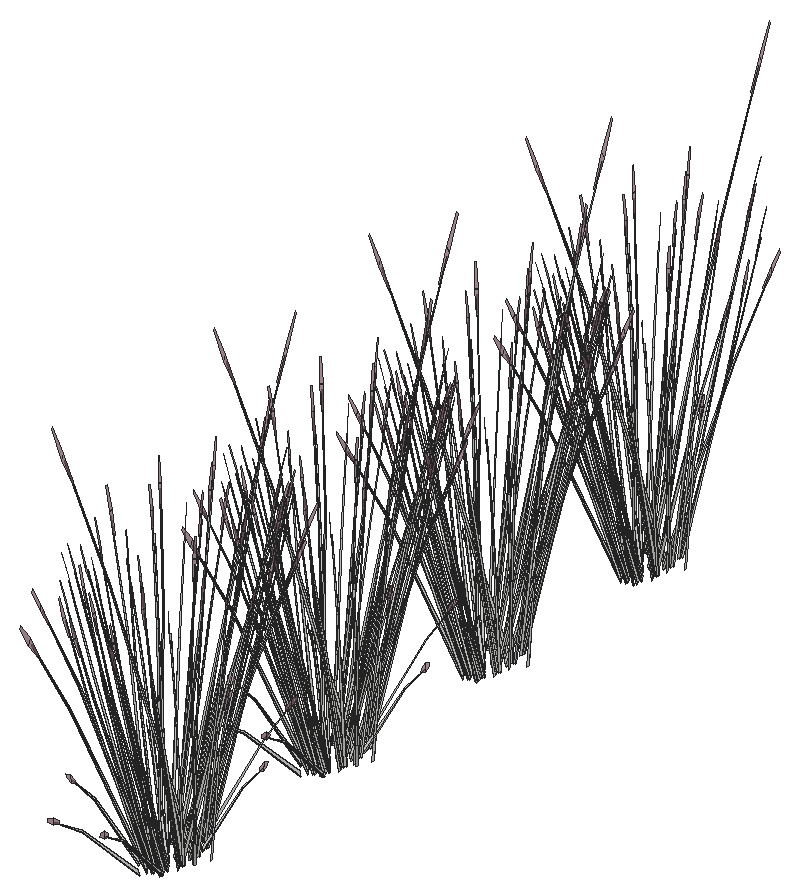
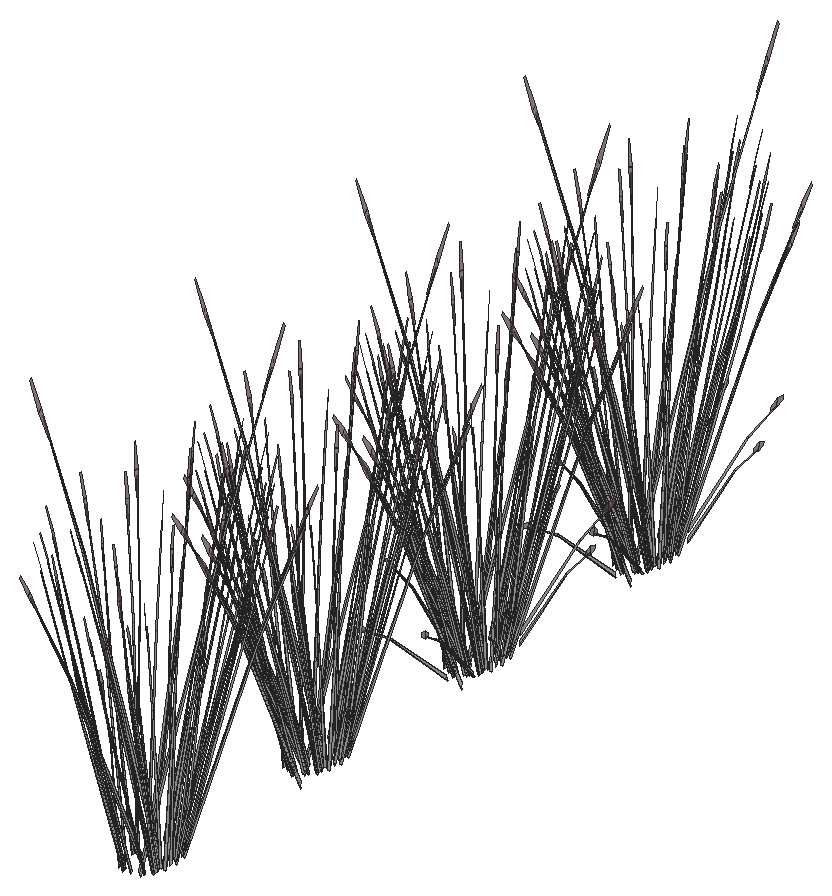
# SketchUp Ruby script. Lengths in inches.
U = 1.inch
M = Sketchup.active_model
def pt(a) = Geom::Point3d.new(a.map { |v| v * U })
def face(e, loops, mat)
  f = e.add_face(loops[0].map { |a| pt(a) })
  loops[1..].each { |l| e.add_face(l.map { |a| pt(a) }).erase! }
  f.material = f.back_material = mat if mat
  f
end
# faces: each face lists its corners as indices into pts; further lists are holes
def faces(e, pts, list, mat = nil) = list.each { |f| face(e, (f[0].is_a?(Array) ? f : [f]).map { |l| l.map { |i| pts[i] } }, mat) }
# xy, xz, yz: faces in a plane at the given z, y or x. An outline is a flat list of corners, or four numbers for a rectangle; further outlines are holes
def ring(l) = l.size == 4 ? [[l[0], l[1]], [l[2], l[1]], [l[2], l[3]], [l[0], l[3]]] : l.each_slice(2).to_a
def flat(e, list, mat, &to3) = list.each { |f| face(e, (f[0].is_a?(Array) ? f : [f]).map { |l| ring(l).map { |u, v| to3.(u, v) } }, mat) }
def xy(e, z, list, mat = nil) = flat(e, list, mat) { |x, y| [x, y, z] }
def xz(e, y, list, mat = nil) = flat(e, list, mat) { |x, z| [x, y, z] }
def yz(e, x, list, mat = nil) = flat(e, list, mat) { |y, z| [x, y, z] }
def lines(e, pts, list) = list.each { |a, b| e.add_line(pt(pts[a]), pt(pts[b])) }
# prism: a flat outline (further loops are holes) pulled along v
def prism(e, loops, v, mat = nil)
  f = face(e, loops, mat); d = Geom::Vector3d.new(v.map { |x| x * U })
  f.pushpull(f.normal.samedirection?(d) ? d.length : -d.length)
end
def box(e, o, s, mat = nil) = prism(e, [[o, [o[0] + s[0], o[1], o[2]], [o[0] + s[0], o[1] + s[1], o[2]], [o[0], o[1] + s[1], o[2]]]], [0, 0, s[2]], mat)
def at(x, y, z, deg = 0) = Geom::Transformation.translation(pt([x, y, z])) * Geom::Transformation.rotation(ORIGIN, Z_AXIS, deg.degrees)
def axes(o, x, y, z) = Geom::Transformation.new([*x, 0, *y, 0, *z, 0, *pt(o).to_a, 1])
def part(name) = M.definitions.add(name)
# library, detail: a bought-in or finely detailed component or shape, given as its bounding box
def library(name, o, s) = part(name).tap { |d| box(d.entities, o, s) }
def detail(e, o, s) = box(e.add_group.entities, o, s)
def put(e, d, t, mat = nil) = e.add_instance(d, t).tap { |i| i.material = mat if mat }
def group(e, t, mat = nil) = e.add_group.tap { |g| g.transformation = t; g.material = mat if mat }.entities
root = M.entities
M.materials.add("LightPink_Translucent").color = [144, 107, 117]
M.materials["LightPink_Translucent"].alpha = 0.75
c1 = part("blade")
p = [[2.15,0.21,22],[0,0.17,0],[0.09,0.45,0],[2.18,0.31,22],[2.29,0.31,22],[0.38,0.45,0],
  [2.48,0.24,33],[2.49,0.24,33],[2.48,0.22,33]]
faces(c1.entities,p,[[0,1,2,3],[4,5,2,3],[6,3,4,7],[8,0,3,6]])
c2 = part("seeds")
p = [[0.3,-0.1,1.38],[-0.01,-0.03,1.59],[-0.01,-0.03,0.03],[0.14,-0.07,-0.07],[0.29,-0.03,3],[0.15,0.01,3.11]]
faces(c2.entities,p,[[0,1,2,3],[1,0,4,5]],"LightPink_Translucent")
c3 = part("blade with seeds")
put(c3.entities,c1,at(0,0,0))
put(c3.entities,c2,axes([2.4,0.25,30.99],[1.5799,-0.05474,1.17369],[-0.12525,1.92788,0.29478],[-0.07173,-0.02425,1.56792]))
put(root,c3,axes([251.1,10.6,2.01],[0.05851,0.19632,1.24382],[-0.27036,0.16528,0.10057],[-0.0611,-0.3082,0.53172]))
put(root,c3,axes([251.55,9.3,2.61],[-0.03915,-0.08573,1.26972],[-0.26126,0.05435,-0.2008],[-0.0417,-0.20505,0.10183]))
put(root,c3,axes([252.72,10.35,2.61],[-0.00247,-0.12169,1.26972],[-0.20868,-0.35171,-0.2008],[0.03226,-0.2132,0.10183]))
put(root,c3,axes([251.84,10.33,2.48],[0.07716,-0.47021,-0.25703],[0.22512,0.13715,0.33183],[-0.02064,-0.18932,0.63492]))
put(root,c3,axes([252.01,10.95,2.01],[-0.04766,0.21017,1.24382],[-0.19993,-0.43493,0.10057],[0.09019,-0.27107,0.53172]))
put(root,c3,axes([251.73,10.65,2.59],[-0.25161,-0.15328,-0.37087],[0.08624,-0.52553,-0.28727],[-0.02307,-0.21159,0.70962]))
put(root,c3,axes([252.27,11.05,2.59],[-0.18323,-0.41084,-0.37087],[0.19356,-0.3598,-0.28727],[0.02788,-0.20874,0.70962]))
put(root,c3,axes([251.94,10.625,2.85],[-0.25047,0.28468,-0.08826],[-0.12309,-0.50526,-0.48986],[-0.03305,-0.21292,0.74434]))
put(root,c3,axes([252.46,11.26,2.85],[-0.2813,-0.0303,-0.08826],[0.00769,-0.57361,-0.48986],[0.01954,-0.22092,0.74434]))
put(root,c3,axes([252.44,10.9,2.48],[0.17318,-0.32193,-0.25703],[0.16394,0.36759,0.33183],[0.02494,-0.18677,0.63492]))
put(root,c3,axes([251.19,10.5,2.48],[-0.03953,-0.49251,-0.25703],[0.22598,-0.13005,0.33183],[-0.0607,-0.14114,0.63492]))
put(root,c3,axes([250.71,11.22,2.01],[0.09507,0.10535,1.24382],[-0.19675,0.44195,0.10057],[-0.12263,-0.19937,0.53172]))
put(root,c3,axes([251.17,10.91,2.59],[-0.25257,0.14535,-0.37087],[-0.04418,-0.55045,-0.28727],[-0.06784,-0.15774,0.70962]))
put(root,c3,axes([252.65,11.99,2.59],[-0.06575,-0.55831,-0.37087],[0.24901,-0.09767,-0.28727],[0.07136,-0.14996,0.70962]))
put(root,c3,axes([250.6875,10.25,2.61],[-0.05507,-0.00432,1.26972],[-0.17533,0.4316,-0.2008],[-0.09355,-0.08819,0.10183]))
put(root,c3,axes([252.77,12.39,2.85],[-0.23676,-0.33715,-0.08826],[0.1364,-0.48826,-0.48986],[0.06689,-0.16972,0.74434]))
put(root,c3,axes([251.79,14.23,1.61],[0.22119,0.24656,1.09782],[-0.21669,0.53118,0.43413],[-0.09706,-0.31482,0.92034]))
put(root,c3,axes([252.84,12.05,2.48],[0.2228,-0.08739,-0.25703],[0.05883,0.49954,0.33183],[0.06385,-0.13418,0.63492]))
put(root,c3,axes([250.67,11.37,2.48],[-0.14563,-0.38283,-0.25703],[0.16629,-0.3624,0.33183],[-0.08449,-0.05514,0.63492]))
put(root,c3,axes([253.48,12.84,2.61],[0.03552,-0.09314,1.26972],[-0.04546,-0.57131,-0.2008],[0.08912,-0.10832,0.10183]))
put(root,c3,axes([250.74,11.75,2.59],[-0.18586,0.40503,-0.37087],[-0.16277,-0.42787,-0.28727],[-0.09443,-0.06163,0.70962]))
put(root,c3,axes([250.84,11.32,2.85],[-0.0137,0.62183,-0.08826],[-0.25949,-0.017,-0.48986],[-0.09994,-0.0432,0.74434]))
put(root,c3,axes([252.78,13.71,2.85],[-0.12878,-0.55367,-0.08826],[0.22857,-0.27208,-0.48986],[0.09632,-0.07305,0.74434]))
put(root,c3,axes([252.77,13.23,2.59],[0.06934,-0.55619,-0.37087],[0.23774,0.19064,-0.28727],[0.09572,-0.051,0.70962]))
put(root,c3,axes([250.51,12.18,2.01],[0.10617,-0.01385,1.24382],[-0.07043,0.60021,0.10057],[-0.1513,-0.03712,0.53172]))
put(root,c3,axes([252.91,13.49,2.48],[0.21272,0.17057,-0.25703],[-0.06204,0.49764,0.33183],[0.08564,-0.04563,0.63492]))
put(root,c3,axes([250.41,12.7,2.48],[-0.21272,-0.17057,-0.25703],[0.06204,-0.49764,0.33183],[-0.08564,0.04563,0.63492]))
put(root,c3,axes([252.33,12.87,2.01],[-0.10617,0.01385,1.24382],[0.07043,-0.60021,0.10057],[0.1513,0.03712,0.53172]))
put(root,c3,axes([251.0625,12.61,1.62],[0.07276,-0.08845,1.2851],[0.02509,0.61759,0.10057],[-0.15759,0.08195,0.4593]))
put(root,c3,axes([250.28,13.03,2.61],[-0.0418,0.07939,1.26972],[0.00356,0.58003,-0.2008],[-0.09581,0.07543,0.10183]))
put(root,c3,axes([250.56,12.95,2.59],[-0.06934,0.55619,-0.37087],[-0.23774,-0.19064,-0.28727],[-0.09572,0.051,0.70962]))
put(root,c3,axes([250.55,12.47,2.85],[0.12878,0.55367,-0.08826],[-0.22857,0.27208,-0.48986],[-0.09632,0.07305,0.74434]))
put(root,c3,axes([253.09,14.875,2.04],[-0.04899,-0.514,-0.02534],[0.23154,-0.11817,-0.1149],[0.04835,0.03259,0.37899]))
put(root,c3,axes([252.49,14.86,2.85],[0.0137,-0.62183,-0.08826],[0.25949,0.017,-0.48986],[0.09994,0.0432,0.74434]))
put(root,c3,axes([252.72,14.49,2.61],[0.05491,-0.01034,1.26972],[0.1506,-0.47504,-0.2008],[0.09767,0.06271,0.10183]))
put(root,c3,axes([250.55,13.24,2.01],[0.08881,-0.12933,1.24382],[0.07477,0.59764,0.10057],[-0.13942,0.13507,0.53172]))
put(root,c3,axes([252.66,14.82,2.48],[0.14563,0.38283,-0.25703],[-0.16629,0.3624,0.33183],[0.08449,0.05514,0.63492]))
put(root,c3,axes([250.49,14.13,2.48],[-0.2228,0.08739,-0.25703],[-0.05883,-0.49954,0.33183],[-0.06385,0.13418,0.63492]))
put(root,c3,axes([252.13,13.84,2.01],[-0.09507,-0.10535,1.24382],[0.19675,-0.44195,0.10057],[0.12263,0.19937,0.53172]))
put(root,c3,axes([252.15,12.45,2.44],[-0.22117,-0.3177,1.00363],[0.23354,-0.49464,0.43304],[0.07136,0.29809,0.97011]))
put(root,c3,axes([250.56,13.79,2.85],[0.23676,0.33715,-0.08826],[-0.1364,0.48826,-0.48986],[-0.06689,0.16972,0.74434]))
put(root,c3,axes([251.98,15.54,2.85],[0.15252,-0.52338,-0.08826],[0.22088,0.30152,-0.48986],[0.07678,0.14787,0.74434]))
put(root,c3,axes([250.875,13.64,2.01],[0.06393,-0.18788,1.24382],[0.16142,0.50711,0.10057],[-0.11071,0.23094,0.53172]))
put(root,c3,axes([250.67,14.1875,2.59],[0.06575,0.55831,-0.37087],[-0.24901,0.09767,-0.28727],[-0.07136,0.14996,0.70962]))
put(root,c3,axes([252.16,15.28,2.59],[0.25257,-0.14535,-0.37087],[0.04418,0.55045,-0.28727],[0.06784,0.15774,0.70962]))
put(root,c3,axes([250.83,14.1,2.01],[0.04766,-0.21017,1.24382],[0.19993,0.43493,0.10057],[-0.09019,0.27107,0.53172]))
put(root,c3,axes([250.88,15.29,2.48],[-0.17318,0.32193,-0.25703],[-0.16394,-0.36759,0.33183],[-0.02494,0.18677,0.63492]))
put(root,c3,axes([250.29,15.19,2.61],[-0.00636,0.121,1.26972],[0.18056,0.42094,-0.2008],[-0.04727,0.19906,0.10183]))
put(root,c3,axes([251.38,15.56,2.85],[0.25047,-0.28468,-0.08826],[0.12309,0.50526,-0.48986],[0.03305,0.21292,0.74434]))
put(root,c3,axes([251.06,15.13,2.83],[0.18323,0.41084,-0.41166],[-0.19356,0.3598,-0.31887],[-0.02788,0.20874,0.78768]))
put(root,c3,axes([251.6,15.53,2.59],[0.25161,0.15328,-0.37087],[-0.08624,0.52553,-0.28727],[0.02307,0.21159,0.70962]))
put(root,c3,axes([251.74,14.45,2.01],[-0.05851,-0.19632,1.24382],[0.27036,-0.16528,0.10057],[0.0611,0.3082,0.53172]))
put(root,c3,axes([251.48,15.85,2.48],[-0.07716,0.47021,-0.25703],[-0.22512,-0.13715,0.33183],[0.02064,0.18932,0.63492]))
put(root,c3,axes([251,14.95,3.07],[-0.00666,0.56559,-0.57235],[-0.28045,-0.03799,0.06907],[-0.0296,0.23961,0.80965]))
put(root,c3,axes([251.26,14.55,2.01],[-0.00626,-0.23468,1.24382],[0.27152,0.15569,0.10057],[-0.01679,0.33444,0.53172]))
put(root,c3,axes([251.32,16.6875,2.61],[0.03244,0.09846,1.26972],[0.26183,0.03868,-0.2008],[0.02633,0.21715,0.10183]))
put(root,c3,axes([250.9,15.74,1.63],[0.00562,-0.31565,1.12021],[0.25293,0.16673,0.1548],[-0.02192,0.33641,0.52896]))
put(root,c3,axes([251.1,27.47,2.01],[0.05851,0.19632,1.24382],[-0.27036,0.16528,0.10057],[-0.0611,-0.3082,0.53172]))
put(root,c3,axes([251.55,26.17,2.61],[-0.03915,-0.08573,1.26972],[-0.26126,0.05435,-0.2008],[-0.0417,-0.20505,0.10183]))
put(root,c3,axes([252.72,27.22,2.61],[-0.00247,-0.12169,1.26972],[-0.20868,-0.35171,-0.2008],[0.03226,-0.2132,0.10183]))
put(root,c3,axes([251.84,27.2,2.48],[0.07716,-0.47021,-0.25703],[0.22512,0.13715,0.33183],[-0.02064,-0.18932,0.63492]))
put(root,c3,axes([252.01,27.82,2.01],[-0.04766,0.21017,1.24382],[-0.19993,-0.43493,0.10057],[0.09019,-0.27107,0.53172]))
put(root,c3,axes([251.73,27.52,2.59],[-0.25161,-0.15328,-0.37087],[0.08624,-0.52553,-0.28727],[-0.02307,-0.21159,0.70962]))
put(root,c3,axes([252.27,27.92,2.59],[-0.18323,-0.41084,-0.37087],[0.19356,-0.3598,-0.28727],[0.02788,-0.20874,0.70962]))
put(root,c3,axes([251.94,27.49,2.85],[-0.25047,0.28468,-0.08826],[-0.12309,-0.50526,-0.48986],[-0.03305,-0.21292,0.74434]))
put(root,c3,axes([252.46,28.13,2.85],[-0.2813,-0.0303,-0.08826],[0.00769,-0.57361,-0.48986],[0.01954,-0.22092,0.74434]))
put(root,c3,axes([252.44,27.76,2.48],[0.17318,-0.32193,-0.25703],[0.16394,0.36759,0.33183],[0.02494,-0.18677,0.63492]))
put(root,c3,axes([251.19,27.37,2.48],[-0.03953,-0.49251,-0.25703],[0.22598,-0.13005,0.33183],[-0.0607,-0.14114,0.63492]))
put(root,c3,axes([250.71,28.08,2.01],[0.09507,0.10535,1.24382],[-0.19675,0.44195,0.10057],[-0.12263,-0.19937,0.53172]))
put(root,c3,axes([251.17,27.77,2.59],[-0.25257,0.14535,-0.37087],[-0.04418,-0.55045,-0.28727],[-0.06784,-0.15774,0.70962]))
put(root,c3,axes([252.65,28.86,2.59],[-0.06575,-0.55831,-0.37087],[0.24901,-0.09767,-0.28727],[0.07136,-0.14996,0.70962]))
put(root,c3,axes([250.6875,27.11,2.61],[-0.05507,-0.00432,1.26972],[-0.17533,0.4316,-0.2008],[-0.09355,-0.08819,0.10183]))
put(root,c3,axes([252.77,29.26,2.85],[-0.23676,-0.33715,-0.08826],[0.1364,-0.48826,-0.48986],[0.06689,-0.16972,0.74434]))
put(root,c3,axes([251.79,31.1,1.61],[0.22119,0.24656,1.09782],[-0.21669,0.53118,0.43413],[-0.09706,-0.31482,0.92034]))
put(root,c3,axes([252.84,28.92,2.48],[0.2228,-0.08739,-0.25703],[0.05883,0.49954,0.33183],[0.06385,-0.13418,0.63492]))
put(root,c3,axes([250.67,28.23,2.48],[-0.14563,-0.38283,-0.25703],[0.16629,-0.3624,0.33183],[-0.08449,-0.05514,0.63492]))
put(root,c3,axes([253.48,29.71,2.61],[0.03552,-0.09314,1.26972],[-0.04546,-0.57131,-0.2008],[0.08912,-0.10832,0.10183]))
put(root,c3,axes([250.74,28.62,2.59],[-0.18586,0.40503,-0.37087],[-0.16277,-0.42787,-0.28727],[-0.09443,-0.06163,0.70962]))
put(root,c3,axes([250.84,28.19,2.85],[-0.0137,0.62183,-0.08826],[-0.25949,-0.017,-0.48986],[-0.09994,-0.0432,0.74434]))
put(root,c3,axes([252.78,30.58,2.85],[-0.12878,-0.55367,-0.08826],[0.22857,-0.27208,-0.48986],[0.09632,-0.07305,0.74434]))
put(root,c3,axes([252.77,30.1,2.59],[0.06934,-0.55619,-0.37087],[0.23774,0.19064,-0.28727],[0.09572,-0.051,0.70962]))
put(root,c3,axes([250.51,29.05,2.01],[0.10617,-0.01385,1.24382],[-0.07043,0.60021,0.10057],[-0.1513,-0.03712,0.53172]))
put(root,c3,axes([252.91,30.36,2.48],[0.21272,0.17057,-0.25703],[-0.06204,0.49764,0.33183],[0.08564,-0.04563,0.63492]))
put(root,c3,axes([250.41,29.5625,2.48],[-0.21272,-0.17057,-0.25703],[0.06204,-0.49764,0.33183],[-0.08564,0.04563,0.63492]))
put(root,c3,axes([252.33,29.74,2.01],[-0.10617,0.01385,1.24382],[0.07043,-0.60021,0.10057],[0.1513,0.03712,0.53172]))
put(root,c3,axes([251.0625,29.48,1.62],[0.07276,-0.08845,1.2851],[0.02509,0.61759,0.10057],[-0.15759,0.08195,0.4593]))
put(root,c3,axes([250.28,29.89,2.61],[-0.0418,0.07939,1.26972],[0.00356,0.58003,-0.2008],[-0.09581,0.07543,0.10183]))
put(root,c3,axes([250.56,29.82,2.59],[-0.06934,0.55619,-0.37087],[-0.23774,-0.19064,-0.28727],[-0.09572,0.051,0.70962]))
put(root,c3,axes([250.55,29.34,2.85],[0.12878,0.55367,-0.08826],[-0.22857,0.27208,-0.48986],[-0.09632,0.07305,0.74434]))
put(root,c3,axes([253.09,31.74,2.04],[-0.04899,-0.514,-0.02534],[0.23154,-0.11817,-0.1149],[0.04835,0.03259,0.37899]))
put(root,c3,axes([252.49,31.73,2.85],[0.0137,-0.62183,-0.08826],[0.25949,0.017,-0.48986],[0.09994,0.0432,0.74434]))
put(root,c3,axes([252.72,31.36,2.61],[0.05491,-0.01034,1.26972],[0.1506,-0.47504,-0.2008],[0.09767,0.06271,0.10183]))
put(root,c3,axes([250.55,30.1,2.01],[0.08881,-0.12933,1.24382],[0.07477,0.59764,0.10057],[-0.13942,0.13507,0.53172]))
put(root,c3,axes([252.66,31.68,2.48],[0.14563,0.38283,-0.25703],[-0.16629,0.3624,0.33183],[0.08449,0.05514,0.63492]))
put(root,c3,axes([250.49,31,2.48],[-0.2228,0.08739,-0.25703],[-0.05883,-0.49954,0.33183],[-0.06385,0.13418,0.63492]))
put(root,c3,axes([252.13,30.7,2.01],[-0.09507,-0.10535,1.24382],[0.19675,-0.44195,0.10057],[0.12263,0.19937,0.53172]))
put(root,c3,axes([252.15,29.32,2.44],[-0.22117,-0.3177,1.00363],[0.23354,-0.49464,0.43304],[0.07136,0.29809,0.97011]))
put(root,c3,axes([250.56,30.66,2.85],[0.23676,0.33715,-0.08826],[-0.1364,0.48826,-0.48986],[-0.06689,0.16972,0.74434]))
put(root,c3,axes([251.98,32.4,2.85],[0.15252,-0.52338,-0.08826],[0.22088,0.30152,-0.48986],[0.07678,0.14787,0.74434]))
put(root,c3,axes([250.875,30.51,2.01],[0.06393,-0.18788,1.24382],[0.16142,0.50711,0.10057],[-0.11071,0.23094,0.53172]))
put(root,c3,axes([250.67,31.06,2.59],[0.06575,0.55831,-0.37087],[-0.24901,0.09767,-0.28727],[-0.07136,0.14996,0.70962]))
put(root,c3,axes([252.16,32.14,2.59],[0.25257,-0.14535,-0.37087],[0.04418,0.55045,-0.28727],[0.06784,0.15774,0.70962]))
put(root,c3,axes([250.83,30.97,2.01],[0.04766,-0.21017,1.24382],[0.19993,0.43493,0.10057],[-0.09019,0.27107,0.53172]))
put(root,c3,axes([250.88,32.15,2.48],[-0.17318,0.32193,-0.25703],[-0.16394,-0.36759,0.33183],[-0.02494,0.18677,0.63492]))
put(root,c3,axes([250.29,32.06,2.61],[-0.00636,0.121,1.26972],[0.18056,0.42094,-0.2008],[-0.04727,0.19906,0.10183]))
put(root,c3,axes([251.38,32.43,2.85],[0.25047,-0.28468,-0.08826],[0.12309,0.50526,-0.48986],[0.03305,0.21292,0.74434]))
put(root,c3,axes([251.06,32,2.83],[0.18323,0.41084,-0.41166],[-0.19356,0.3598,-0.31887],[-0.02788,0.20874,0.78768]))
put(root,c3,axes([251.6,32.4,2.59],[0.25161,0.15328,-0.37087],[-0.08624,0.52553,-0.28727],[0.02307,0.21159,0.70962]))
put(root,c3,axes([251.74,31.32,2.01],[-0.05851,-0.19632,1.24382],[0.27036,-0.16528,0.10057],[0.0611,0.3082,0.53172]))
put(root,c3,axes([251.48,32.72,2.48],[-0.07716,0.47021,-0.25703],[-0.22512,-0.13715,0.33183],[0.02064,0.18932,0.63492]))
put(root,c3,axes([251,31.81,3.07],[-0.00666,0.56559,-0.57235],[-0.28045,-0.03799,0.06907],[-0.0296,0.23961,0.80965]))
put(root,c3,axes([251.26,31.41,2.01],[-0.00626,-0.23468,1.24382],[0.27152,0.15569,0.10057],[-0.01679,0.33444,0.53172]))
put(root,c3,axes([251.32,33.56,2.61],[0.03244,0.09846,1.26972],[0.26183,0.03868,-0.2008],[0.02633,0.21715,0.10183]))
put(root,c3,axes([250.9,32.61,1.63],[0.00562,-0.31565,1.12021],[0.25293,0.16673,0.1548],[-0.02192,0.33641,0.52896]))
put(root,c3,axes([251.1,43.625,2.01],[0.05851,0.19632,1.24382],[-0.27036,0.16528,0.10057],[-0.0611,-0.3082,0.53172]))
put(root,c3,axes([251.84,43.35,2.48],[0.07716,-0.47021,-0.25703],[0.22512,0.13715,0.33183],[-0.02064,-0.18932,0.63492]))
put(root,c3,axes([252.01,43.97,2.01],[-0.04766,0.21017,1.24382],[-0.19993,-0.43493,0.10057],[0.09019,-0.27107,0.53172]))
put(root,c3,axes([251.73,43.67,2.59],[-0.25161,-0.15328,-0.37087],[0.08624,-0.52553,-0.28727],[-0.02307,-0.21159,0.70962]))
put(root,c3,axes([252.27,44.07,2.59],[-0.18323,-0.41084,-0.37087],[0.19356,-0.3598,-0.28727],[0.02788,-0.20874,0.70962]))
put(root,c3,axes([251.94,43.65,2.85],[-0.25047,0.28468,-0.08826],[-0.12309,-0.50526,-0.48986],[-0.03305,-0.21292,0.74434]))
put(root,c3,axes([252.46,44.29,2.85],[-0.2813,-0.0303,-0.08826],[0.00769,-0.57361,-0.48986],[0.01954,-0.22092,0.74434]))
put(root,c3,axes([252.44,43.92,2.48],[0.17318,-0.32193,-0.25703],[0.16394,0.36759,0.33183],[0.02494,-0.18677,0.63492]))
put(root,c3,axes([251.19,43.52,2.48],[-0.03953,-0.49251,-0.25703],[0.22598,-0.13005,0.33183],[-0.0607,-0.14114,0.63492]))
put(root,c3,axes([250.71,44.24,2.01],[0.09507,0.10535,1.24382],[-0.19675,0.44195,0.10057],[-0.12263,-0.19937,0.53172]))
put(root,c3,axes([251.17,43.93,2.59],[-0.25257,0.14535,-0.37087],[-0.04418,-0.55045,-0.28727],[-0.06784,-0.15774,0.70962]))
put(root,c3,axes([252.65,45.01,2.59],[-0.06575,-0.55831,-0.37087],[0.24901,-0.09767,-0.28727],[0.07136,-0.14996,0.70962]))
put(root,c3,axes([252.77,45.41,2.85],[-0.23676,-0.33715,-0.08826],[0.1364,-0.48826,-0.48986],[0.06689,-0.16972,0.74434]))
put(root,c3,axes([251.79,47.26,1.61],[0.22119,0.24656,1.09782],[-0.21669,0.53118,0.43413],[-0.09706,-0.31482,0.92034]))
put(root,c3,axes([252.84,45.07,2.48],[0.2228,-0.08739,-0.25703],[0.05883,0.49954,0.33183],[0.06385,-0.13418,0.63492]))
put(root,c3,axes([250.67,44.39,2.48],[-0.14563,-0.38283,-0.25703],[0.16629,-0.3624,0.33183],[-0.08449,-0.05514,0.63492]))
put(root,c3,axes([250.74,44.77,2.59],[-0.18586,0.40503,-0.37087],[-0.16277,-0.42787,-0.28727],[-0.09443,-0.06163,0.70962]))
put(root,c3,axes([250.84,44.34,2.85],[-0.0137,0.62183,-0.08826],[-0.25949,-0.017,-0.48986],[-0.09994,-0.0432,0.74434]))
put(root,c3,axes([252.78,46.73,2.85],[-0.12878,-0.55367,-0.08826],[0.22857,-0.27208,-0.48986],[0.09632,-0.07305,0.74434]))
put(root,c3,axes([252.77,46.25,2.59],[0.06934,-0.55619,-0.37087],[0.23774,0.19064,-0.28727],[0.09572,-0.051,0.70962]))
put(root,c3,axes([250.51,45.2,2.01],[0.10617,-0.01385,1.24382],[-0.07043,0.60021,0.10057],[-0.1513,-0.03712,0.53172]))
put(root,c3,axes([252.91,46.51,2.48],[0.21272,0.17057,-0.25703],[-0.06204,0.49764,0.33183],[0.08564,-0.04563,0.63492]))
put(root,c3,axes([250.41,45.72,2.48],[-0.21272,-0.17057,-0.25703],[0.06204,-0.49764,0.33183],[-0.08564,0.04563,0.63492]))
put(root,c3,axes([252.33,45.89,2.01],[-0.10617,0.01385,1.24382],[0.07043,-0.60021,0.10057],[0.1513,0.03712,0.53172]))
put(root,c3,axes([251.0625,45.63,1.62],[0.07276,-0.08845,1.2851],[0.02509,0.61759,0.10057],[-0.15759,0.08195,0.4593]))
put(root,c3,axes([250.28,46.05,2.61],[-0.0418,0.07939,1.26972],[0.00356,0.58003,-0.2008],[-0.09581,0.07543,0.10183]))
put(root,c3,axes([250.56,45.97,2.59],[-0.06934,0.55619,-0.37087],[-0.23774,-0.19064,-0.28727],[-0.09572,0.051,0.70962]))
put(root,c3,axes([250.55,45.49,2.85],[0.12878,0.55367,-0.08826],[-0.22857,0.27208,-0.48986],[-0.09632,0.07305,0.74434]))
put(root,c3,axes([253.09,47.9,2.04],[-0.04899,-0.514,-0.02534],[0.23154,-0.11817,-0.1149],[0.04835,0.03259,0.37899]))
put(root,c3,axes([252.49,47.88,2.85],[0.0137,-0.62183,-0.08826],[0.25949,0.017,-0.48986],[0.09994,0.0432,0.74434]))
put(root,c3,axes([250.55,46.26,2.01],[0.08881,-0.12933,1.24382],[0.07477,0.59764,0.10057],[-0.13942,0.13507,0.53172]))
put(root,c3,axes([252.66,47.84,2.48],[0.14563,0.38283,-0.25703],[-0.16629,0.3624,0.33183],[0.08449,0.05514,0.63492]))
put(root,c3,axes([250.49,47.15,2.48],[-0.2228,0.08739,-0.25703],[-0.05883,-0.49954,0.33183],[-0.06385,0.13418,0.63492]))
put(root,c3,axes([252.13,46.86,2.01],[-0.09507,-0.10535,1.24382],[0.19675,-0.44195,0.10057],[0.12263,0.19937,0.53172]))
put(root,c3,axes([252.15,45.47,2.44],[-0.22117,-0.3177,1.00363],[0.23354,-0.49464,0.43304],[0.07136,0.29809,0.97011]))
put(root,c3,axes([250.56,46.81,2.85],[0.23676,0.33715,-0.08826],[-0.1364,0.48826,-0.48986],[-0.06689,0.16972,0.74434]))
put(root,c3,axes([251.98,48.56,2.85],[0.15252,-0.52338,-0.08826],[0.22088,0.30152,-0.48986],[0.07678,0.14787,0.74434]))
put(root,c3,axes([250.875,46.66,2.01],[0.06393,-0.18788,1.24382],[0.16142,0.50711,0.10057],[-0.11071,0.23094,0.53172]))
put(root,c3,axes([250.67,47.21,2.59],[0.06575,0.55831,-0.37087],[-0.24901,0.09767,-0.28727],[-0.07136,0.14996,0.70962]))
put(root,c3,axes([252.16,48.3,2.59],[0.25257,-0.14535,-0.37087],[0.04418,0.55045,-0.28727],[0.06784,0.15774,0.70962]))
put(root,c3,axes([250.83,47.12,2.01],[0.04766,-0.21017,1.24382],[0.19993,0.43493,0.10057],[-0.09019,0.27107,0.53172]))
put(root,c3,axes([250.88,48.31,2.48],[-0.17318,0.32193,-0.25703],[-0.16394,-0.36759,0.33183],[-0.02494,0.18677,0.63492]))
put(root,c3,axes([251.38,48.58,2.85],[0.25047,-0.28468,-0.08826],[0.12309,0.50526,-0.48986],[0.03305,0.21292,0.74434]))
put(root,c3,axes([251.06,48.15,2.83],[0.18323,0.41084,-0.41166],[-0.19356,0.3598,-0.31887],[-0.02788,0.20874,0.78768]))
put(root,c3,axes([251.6,48.55,2.59],[0.25161,0.15328,-0.37087],[-0.08624,0.52553,-0.28727],[0.02307,0.21159,0.70962]))
put(root,c3,axes([251.74,47.47,2.01],[-0.05851,-0.19632,1.24382],[0.27036,-0.16528,0.10057],[0.0611,0.3082,0.53172]))
put(root,c3,axes([251.48,48.875,2.48],[-0.07716,0.47021,-0.25703],[-0.22512,-0.13715,0.33183],[0.02064,0.18932,0.63492]))
put(root,c3,axes([251,47.97,3.07],[-0.00666,0.56559,-0.57235],[-0.28045,-0.03799,0.06907],[-0.0296,0.23961,0.80965]))
put(root,c3,axes([251.26,47.57,2.01],[-0.00626,-0.23468,1.24382],[0.27152,0.15569,0.10057],[-0.01679,0.33444,0.53172]))
put(root,c3,axes([250.9,48.76,1.63],[0.00562,-0.31565,1.12021],[0.25293,0.16673,0.1548],[-0.02192,0.33641,0.52896]))
put(root,c3,axes([251.1,60.07,2.01],[0.05851,0.19632,1.24382],[-0.27036,0.16528,0.10057],[-0.0611,-0.3082,0.53172]))
put(root,c3,axes([251.84,59.8,2.48],[0.07716,-0.47021,-0.25703],[0.22512,0.13715,0.33183],[-0.02064,-0.18932,0.63492]))
put(root,c3,axes([252.01,60.42,2.01],[-0.04766,0.21017,1.24382],[-0.19993,-0.43493,0.10057],[0.09019,-0.27107,0.53172]))
put(root,c3,axes([251.73,60.12,2.59],[-0.25161,-0.15328,-0.37087],[0.08624,-0.52553,-0.28727],[-0.02307,-0.21159,0.70962]))
put(root,c3,axes([252.27,60.52,2.59],[-0.18323,-0.41084,-0.37087],[0.19356,-0.3598,-0.28727],[0.02788,-0.20874,0.70962]))
put(root,c3,axes([251.94,60.1,2.85],[-0.25047,0.28468,-0.08826],[-0.12309,-0.50526,-0.48986],[-0.03305,-0.21292,0.74434]))
put(root,c3,axes([252.46,60.74,2.85],[-0.2813,-0.0303,-0.08826],[0.00769,-0.57361,-0.48986],[0.01954,-0.22092,0.74434]))
put(root,c3,axes([252.44,60.37,2.48],[0.17318,-0.32193,-0.25703],[0.16394,0.36759,0.33183],[0.02494,-0.18677,0.63492]))
put(root,c3,axes([251.19,59.97,2.48],[-0.03953,-0.49251,-0.25703],[0.22598,-0.13005,0.33183],[-0.0607,-0.14114,0.63492]))
put(root,c3,axes([250.71,60.6875,2.01],[0.09507,0.10535,1.24382],[-0.19675,0.44195,0.10057],[-0.12263,-0.19937,0.53172]))
put(root,c3,axes([251.17,60.38,2.59],[-0.25257,0.14535,-0.37087],[-0.04418,-0.55045,-0.28727],[-0.06784,-0.15774,0.70962]))
put(root,c3,axes([252.65,61.47,2.59],[-0.06575,-0.55831,-0.37087],[0.24901,-0.09767,-0.28727],[0.07136,-0.14996,0.70962]))
put(root,c3,axes([252.77,61.86,2.85],[-0.23676,-0.33715,-0.08826],[0.1364,-0.48826,-0.48986],[0.06689,-0.16972,0.74434]))
put(root,c3,axes([251.79,63.71,1.61],[0.22119,0.24656,1.09782],[-0.21669,0.53118,0.43413],[-0.09706,-0.31482,0.92034]))
put(root,c3,axes([252.84,61.52,2.48],[0.2228,-0.08739,-0.25703],[0.05883,0.49954,0.33183],[0.06385,-0.13418,0.63492]))
put(root,c3,axes([250.67,60.84,2.48],[-0.14563,-0.38283,-0.25703],[0.16629,-0.3624,0.33183],[-0.08449,-0.05514,0.63492]))
put(root,c3,axes([250.74,61.22,2.59],[-0.18586,0.40503,-0.37087],[-0.16277,-0.42787,-0.28727],[-0.09443,-0.06163,0.70962]))
put(root,c3,axes([250.84,60.79,2.85],[-0.0137,0.62183,-0.08826],[-0.25949,-0.017,-0.48986],[-0.09994,-0.0432,0.74434]))
put(root,c3,axes([252.78,63.18,2.85],[-0.12878,-0.55367,-0.08826],[0.22857,-0.27208,-0.48986],[0.09632,-0.07305,0.74434]))
put(root,c3,axes([252.77,62.71,2.59],[0.06934,-0.55619,-0.37087],[0.23774,0.19064,-0.28727],[0.09572,-0.051,0.70962]))
put(root,c3,axes([250.51,61.65,2.01],[0.10617,-0.01385,1.24382],[-0.07043,0.60021,0.10057],[-0.1513,-0.03712,0.53172]))
put(root,c3,axes([252.91,62.96,2.48],[0.21272,0.17057,-0.25703],[-0.06204,0.49764,0.33183],[0.08564,-0.04563,0.63492]))
put(root,c3,axes([250.41,62.17,2.48],[-0.21272,-0.17057,-0.25703],[0.06204,-0.49764,0.33183],[-0.08564,0.04563,0.63492]))
put(root,c3,axes([252.33,62.34,2.01],[-0.10617,0.01385,1.24382],[0.07043,-0.60021,0.10057],[0.1513,0.03712,0.53172]))
put(root,c3,axes([251.0625,62.08,1.62],[0.07276,-0.08845,1.2851],[0.02509,0.61759,0.10057],[-0.15759,0.08195,0.4593]))
put(root,c3,axes([250.56,62.42,2.59],[-0.06934,0.55619,-0.37087],[-0.23774,-0.19064,-0.28727],[-0.09572,0.051,0.70962]))
put(root,c3,axes([250.55,61.94,2.85],[0.12878,0.55367,-0.08826],[-0.22857,0.27208,-0.48986],[-0.09632,0.07305,0.74434]))
put(root,c3,axes([253.09,64.35,2.04],[-0.04899,-0.514,-0.02534],[0.23154,-0.11817,-0.1149],[0.04835,0.03259,0.37899]))
put(root,c3,axes([252.49,64.33,2.85],[0.0137,-0.62183,-0.08826],[0.25949,0.017,-0.48986],[0.09994,0.0432,0.74434]))
put(root,c3,axes([250.55,62.71,2.01],[0.08881,-0.12933,1.24382],[0.07477,0.59764,0.10057],[-0.13942,0.13507,0.53172]))
put(root,c3,axes([252.66,64.29,2.48],[0.14563,0.38283,-0.25703],[-0.16629,0.3624,0.33183],[0.08449,0.05514,0.63492]))
put(root,c3,axes([250.49,63.6,2.48],[-0.2228,0.08739,-0.25703],[-0.05883,-0.49954,0.33183],[-0.06385,0.13418,0.63492]))
put(root,c3,axes([252.13,63.31,2.01],[-0.09507,-0.10535,1.24382],[0.19675,-0.44195,0.10057],[0.12263,0.19937,0.53172]))
put(root,c3,axes([252.15,61.92,2.44],[-0.22117,-0.3177,1.00363],[0.23354,-0.49464,0.43304],[0.07136,0.29809,0.97011]))
put(root,c3,axes([250.56,63.26,2.85],[0.23676,0.33715,-0.08826],[-0.1364,0.48826,-0.48986],[-0.06689,0.16972,0.74434]))
put(root,c3,axes([251.98,65.01,2.85],[0.15252,-0.52338,-0.08826],[0.22088,0.30152,-0.48986],[0.07678,0.14787,0.74434]))
put(root,c3,axes([250.875,63.11,2.01],[0.06393,-0.18788,1.24382],[0.16142,0.50711,0.10057],[-0.11071,0.23094,0.53172]))
put(root,c3,axes([250.67,63.66,2.59],[0.06575,0.55831,-0.37087],[-0.24901,0.09767,-0.28727],[-0.07136,0.14996,0.70962]))
put(root,c3,axes([252.16,64.75,2.59],[0.25257,-0.14535,-0.37087],[0.04418,0.55045,-0.28727],[0.06784,0.15774,0.70962]))
put(root,c3,axes([250.83,63.57,2.01],[0.04766,-0.21017,1.24382],[0.19993,0.43493,0.10057],[-0.09019,0.27107,0.53172]))
put(root,c3,axes([250.88,64.76,2.48],[-0.17318,0.32193,-0.25703],[-0.16394,-0.36759,0.33183],[-0.02494,0.18677,0.63492]))
put(root,c3,axes([251.38,65.03,2.85],[0.25047,-0.28468,-0.08826],[0.12309,0.50526,-0.48986],[0.03305,0.21292,0.74434]))
